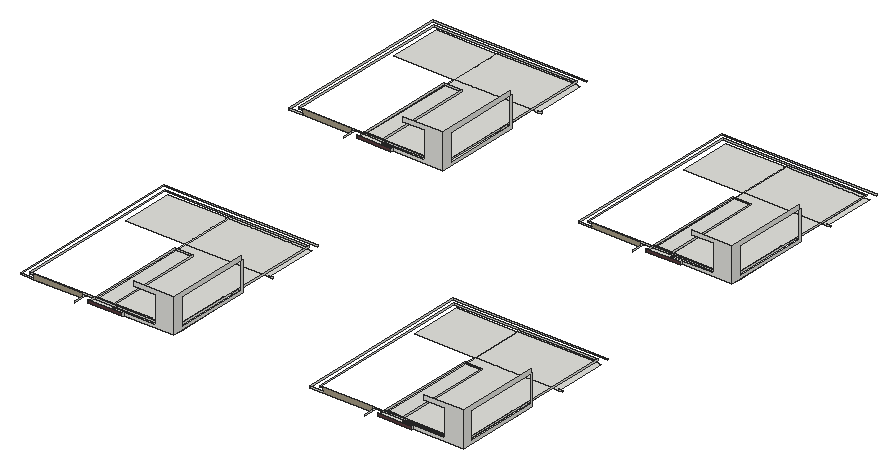
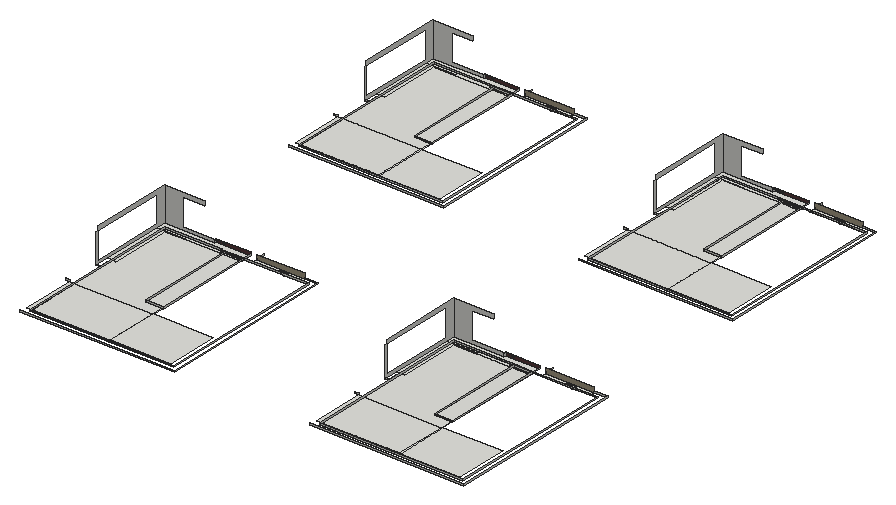
# SketchUp Ruby script. Lengths in inches.
U = 1.inch
M = Sketchup.active_model
def pt(a) = Geom::Point3d.new(a.map { |v| v * U })
def face(e, loops, mat)
  f = e.add_face(loops[0].map { |a| pt(a) })
  loops[1..].each { |l| e.add_face(l.map { |a| pt(a) }).erase! }
  f.material = f.back_material = mat if mat
  f
end
# faces: each face lists its corners as indices into pts; further lists are holes
def faces(e, pts, list, mat = nil) = list.each { |f| face(e, (f[0].is_a?(Array) ? f : [f]).map { |l| l.map { |i| pts[i] } }, mat) }
# xy, xz, yz: faces in a plane at the given z, y or x. An outline is a flat list of corners, or four numbers for a rectangle; further outlines are holes
def ring(l) = l.size == 4 ? [[l[0], l[1]], [l[2], l[1]], [l[2], l[3]], [l[0], l[3]]] : l.each_slice(2).to_a
def flat(e, list, mat, &to3) = list.each { |f| face(e, (f[0].is_a?(Array) ? f : [f]).map { |l| ring(l).map { |u, v| to3.(u, v) } }, mat) }
def xy(e, z, list, mat = nil) = flat(e, list, mat) { |x, y| [x, y, z] }
def xz(e, y, list, mat = nil) = flat(e, list, mat) { |x, z| [x, y, z] }
def yz(e, x, list, mat = nil) = flat(e, list, mat) { |y, z| [x, y, z] }
def lines(e, pts, list) = list.each { |a, b| e.add_line(pt(pts[a]), pt(pts[b])) }
# prism: a flat outline (further loops are holes) pulled along v
def prism(e, loops, v, mat = nil)
  f = face(e, loops, mat); d = Geom::Vector3d.new(v.map { |x| x * U })
  f.pushpull(f.normal.samedirection?(d) ? d.length : -d.length)
end
def box(e, o, s, mat = nil) = prism(e, [[o, [o[0] + s[0], o[1], o[2]], [o[0] + s[0], o[1] + s[1], o[2]], [o[0], o[1] + s[1], o[2]]]], [0, 0, s[2]], mat)
def at(x, y, z, deg = 0) = Geom::Transformation.translation(pt([x, y, z])) * Geom::Transformation.rotation(ORIGIN, Z_AXIS, deg.degrees)
def axes(o, x, y, z) = Geom::Transformation.new([*x, 0, *y, 0, *z, 0, *pt(o).to_a, 1])
def part(name) = M.definitions.add(name)
# library, detail: a bought-in or finely detailed component or shape, given as its bounding box
def library(name, o, s) = part(name).tap { |d| box(d.entities, o, s) }
def detail(e, o, s) = box(e.add_group.entities, o, s)
def put(e, d, t, mat = nil) = e.add_instance(d, t).tap { |i| i.material = mat if mat }
def group(e, t, mat = nil) = e.add_group.tap { |g| g.transformation = t; g.material = mat if mat }.entities
root = M.entities
M.materials.add("[Concrete Tile]").color = [165, 155, 133]
M.materials.add("[Granite Brown]").color = [89, 59, 61]
xy(root,504,[[557.88,1788.5,557.88,1822.9375,890.875,1822.9375,890.875,1835.1875,913.875,1835.1875,913.875,1795.6875,701.53,1795.6875,701.53,1788.5],[1776.07,1788.5,1776.07,1822.9375,2109.0625,1822.9375,2109.0625,1835.1875,2132.0625,1835.1875,2132.0625,1795.6875,1919.71,1795.6875,1919.71,1788.5],[319.53,1799.9375,319.53,1822.9375,401.14,1822.9375,401.14,1806.5625,431.33,1806.5625,431.33,1822.9375,523.04,1822.9375,523.04,1799.9375],[1537.72,1799.9375,1537.72,1822.9375,1619.33,1822.9375,1619.33,1806.5625,1649.52,1806.5625,1649.52,1822.9375,1741.23,1822.9375,1741.23,1799.9375],[557.4,1822.9375,557.4,1827.68,556.44,1827.91,555.39,1823.41],
  [557.4,1822.9375,557.88,1825,557.88,1827.4375,557.4,1827.4375],[650.48,1822.9375,890.875,1822.9375,890.875,1835.1875,784.3125,1835.1875,784.3125,1837.8125,632.49,1837.8125,632.49,1827.4375,650.48,1827.4375],[648.79,1822.9375,650.48,1827.4375],[1775.59,1822.9375,1775.59,1827.68,1774.63,1827.91,1773.58,1823.41],[1775.59,1822.9375,1776.07,1825,1776.07,1827.4375,1775.59,1827.4375],
  [1868.66,1822.9375,2109.0625,1822.9375,2109.0625,1835.1875,2002.5,1835.1875,2002.5,1837.8125,1850.67,1837.8125,1850.67,1827.4375,1868.66,1827.4375],[1866.98,1822.9375,1868.66,1827.4375],[557.88,1825,558.45,1827.4375,557.88,1827.4375],[1776.07,1825,1776.64,1827.4375,1776.07,1827.4375],[557.4,1827.4375,557.88,1827.4375,557.88,1827.57,557.4,1827.68],
  [557.88,1827.4375,558.45,1827.4375,557.88,1827.57],[558.45,1827.4375,558.96,1829.625,557.88,1829.625,557.88,1827.57],[558.45,1827.4375,558.96,1829.625,560,1829.625,560,1827.4375],[560,1827.4375,564.5,1829.625],[564.5,1827.4375,632.49,1829.625],
  [1775.59,1827.4375,1776.07,1827.4375,1776.07,1827.57,1775.59,1827.68],[1776.07,1827.4375,1776.64,1827.4375,1776.07,1827.57],[1776.64,1827.4375,1777.15,1829.625,1776.07,1829.625,1776.07,1827.57],[1776.64,1827.4375,1777.15,1829.625,1778.1875,1829.625,1778.1875,1827.4375],[1778.1875,1827.4375,1782.6875,1829.625],
  [1782.6875,1827.4375,1850.67,1829.625],[557.88,1827.57,557.88,1827.68,557.4,1827.68],[1776.07,1827.57,1776.07,1827.68,1775.59,1827.68],[557.4,1827.68,557.4,1829.99,556.96,1830.09,556.44,1827.91],[1775.59,1827.68,1775.59,1829.99,1775.14,1830.09,1774.63,1827.91],
  [557.4,1829.625,557.88,1829.625,557.88,1829.875,557.4,1829.99],[557.88,1829.625,557.88,1829.875,558.96,1829.625],[558.96,1829.625,557.88,1829.875,557.88,1834.0625,557.99,1834.53,560,1834.0625],[558.96,1829.625,560,1834.0625,560,1829.625],[560,1829.625,564.5,1834.0625],
  [564.5,1829.625,632.49,1837.8125],[1775.59,1829.625,1776.07,1829.625,1776.07,1829.875,1775.59,1829.99],[1776.07,1829.625,1776.07,1829.875,1777.15,1829.625],[1777.15,1829.625,1776.07,1829.875,1776.07,1834.0625,1776.18,1834.53,1778.1875,1834.0625],[1777.15,1829.625,1778.1875,1834.0625,1778.1875,1829.625],
  [1778.1875,1829.625,1782.6875,1834.0625],[1782.6875,1829.625,1850.67,1837.8125],[557.4,1829.99,557.4,1832,556.96,1830.09],[1775.59,1829.99,1775.59,1832,1775.14,1830.09],[557.4,1832,557.88,1834.0625,557.88,1832],
  [557.4,1832,557.88,1834.0625,557.88,1837.8125,557.4,1837.8125],[1775.59,1832,1776.07,1834.0625,1776.07,1832],[1775.59,1832,1776.07,1834.0625,1776.07,1837.8125,1775.59,1837.8125],[557.88,1834.0625,557.88,1837.8125,560,1837.8125,560,1834.0625,557.99,1834.53],[560,1834.0625,564.5,1837.8125],
  [1776.07,1834.0625,1776.07,1837.8125,1778.1875,1837.8125,1778.1875,1834.0625,1776.18,1834.53],[1778.1875,1834.0625,1782.6875,1837.8125],[784.3125,1835.1875,890.875,1835.1875,890.875,2095.79,878.5625,2095.79,878.5625,1837.8125,784.3125,1837.8125],[890.875,1835.1875,913.875,2095.79],[2002.5,1835.1875,2109.0625,1835.1875,2109.0625,2095.79,2096.75,2095.79,2096.75,1837.8125,2002.5,1837.8125],
  [2109.0625,1835.1875,2132.0625,2095.79],[557.4,1837.8125,560,2246.6875],[560,1837.8125,564.5,1838.5625],[564.5,1837.8125,632.49,2246.6875],[632.49,1837.8125,878.5625,1837.8125,878.5625,2095.79,890.875,2095.79,890.875,2295.875,564.5,2295.875,564.5,2246.6875,632.49,2246.6875],
  [1775.59,1837.8125,1778.1875,2246.6875],[1778.1875,1837.8125,1782.6875,1838.5625],[1782.6875,1837.8125,1850.67,2246.6875],[1850.67,1837.8125,2096.75,1837.8125,2096.75,2095.79,2109.0625,2095.79,2109.0625,2295.875,1782.6875,2295.875,1782.6875,2246.6875,1850.67,2246.6875],[560,1838.5625,564.5,2246.6875],
  [1778.1875,1838.5625,1782.6875,2246.6875],[560,2246.6875,564.5,2295.875],[1778.1875,2246.6875,1782.6875,2295.875],[308.87,2295.875,560,2518.89],[560,2295.875,564.5,2518.89],
  [564.5,2295.875,890.875,2518.89],[890.875,2295.875,913.875,2518.89],[1527.06,2295.875,1778.1875,2518.89],[1778.1875,2295.875,1782.6875,2518.89],[1782.6875,2295.875,2109.0625,2518.89],
  [2109.0625,2295.875,2132.0625,2518.89],[560,2518.89,564.5,2531.375],[564.5,2518.89,890.875,2531.375],[1778.1875,2518.89,1782.6875,2531.375],[1782.6875,2518.89,2109.0625,2531.375],
  [557.88,3203.1875,557.88,3237.625,890.875,3237.625,890.875,3249.875,913.875,3249.875,913.875,3210.375,701.53,3210.375,701.53,3203.1875],[1776.07,3203.1875,1776.07,3237.625,2109.0625,3237.625,2109.0625,3249.875,2132.0625,3249.875,2132.0625,3210.375,1919.71,3210.375,1919.71,3203.1875],[319.53,3214.625,319.53,3237.625,401.14,3237.625,401.14,3221.25,431.33,3221.25,431.33,3237.625,523.04,3237.625,523.04,3214.625],[1537.72,3214.625,1537.72,3237.625,1619.33,3237.625,1619.33,3221.25,1649.52,3221.25,1649.52,3237.625,1741.23,3237.625,1741.23,3214.625],[557.4,3237.625,557.4,3242.37,556.44,3242.59,555.39,3238.09],
  [557.4,3237.625,557.88,3239.6875,557.88,3242.125,557.4,3242.125],[650.48,3237.625,890.875,3237.625,890.875,3249.875,784.3125,3249.875,784.3125,3252.5,632.49,3252.5,632.49,3242.125,650.48,3242.125],[648.79,3237.625,650.48,3242.125],[1775.59,3237.625,1775.59,3242.37,1774.63,3242.59,1773.58,3238.09],[1775.59,3237.625,1776.07,3239.6875,1776.07,3242.125,1775.59,3242.125],
  [1868.66,3237.625,2109.0625,3237.625,2109.0625,3249.875,2002.5,3249.875,2002.5,3252.5,1850.67,3252.5,1850.67,3242.125,1868.66,3242.125],[1866.98,3237.625,1868.66,3242.125],[557.88,3239.6875,558.45,3242.125,557.88,3242.125],[1776.07,3239.6875,1776.64,3242.125,1776.07,3242.125],[557.4,3242.125,557.88,3242.125,557.88,3242.26,557.4,3242.37],
  [557.88,3242.125,558.45,3242.125,557.88,3242.26],[558.45,3242.125,558.96,3244.3125,557.88,3244.3125,557.88,3242.26],[558.45,3242.125,558.96,3244.3125,560,3244.3125,560,3242.125],[560,3242.125,564.5,3244.3125],[564.5,3242.125,632.49,3244.3125],
  [1775.59,3242.125,1776.07,3242.125,1776.07,3242.26,1775.59,3242.37],[1776.07,3242.125,1776.64,3242.125,1776.07,3242.26],[1776.64,3242.125,1777.15,3244.3125,1776.07,3244.3125,1776.07,3242.26],[1776.64,3242.125,1777.15,3244.3125,1778.1875,3244.3125,1778.1875,3242.125],[1778.1875,3242.125,1782.6875,3244.3125],
  [1782.6875,3242.125,1850.67,3244.3125],[557.88,3242.26,557.88,3242.37,557.4,3242.37],[1776.07,3242.26,1776.07,3242.37,1775.59,3242.37],[557.4,3242.37,557.4,3244.68,556.96,3244.78,556.44,3242.59],[1775.59,3242.37,1775.59,3244.68,1775.14,3244.78,1774.63,3242.59],
  [557.4,3244.3125,557.88,3244.3125,557.88,3244.5625,557.4,3244.68],[557.88,3244.3125,557.88,3244.5625,558.96,3244.3125],[558.96,3244.3125,557.88,3244.5625,557.88,3248.75,557.99,3249.22,560,3248.75],[558.96,3244.3125,560,3248.75,560,3244.3125],[560,3244.3125,564.5,3248.75],
  [564.5,3244.3125,632.49,3252.5],[1775.59,3244.3125,1776.07,3244.3125,1776.07,3244.5625,1775.59,3244.68],[1776.07,3244.3125,1776.07,3244.5625,1777.15,3244.3125],[1777.15,3244.3125,1776.07,3244.5625,1776.07,3248.75,1776.18,3249.22,1778.1875,3248.75],[1777.15,3244.3125,1778.1875,3248.75,1778.1875,3244.3125],
  [1778.1875,3244.3125,1782.6875,3248.75],[1782.6875,3244.3125,1850.67,3252.5],[557.4,3244.68,557.4,3246.6875,556.96,3244.78],[1775.59,3244.68,1775.59,3246.6875,1775.14,3244.78],[557.4,3246.6875,557.88,3248.75,557.88,3246.6875],
  [557.4,3246.6875,557.88,3248.75,557.88,3252.5,557.4,3252.5],[1775.59,3246.6875,1776.07,3248.75,1776.07,3246.6875],[1775.59,3246.6875,1776.07,3248.75,1776.07,3252.5,1775.59,3252.5],[557.88,3248.75,557.88,3252.5,560,3252.5,560,3248.75,557.99,3249.22],[560,3248.75,564.5,3252.5],
  [1776.07,3248.75,1776.07,3252.5,1778.1875,3252.5,1778.1875,3248.75,1776.18,3249.22],[1778.1875,3248.75,1782.6875,3252.5],[784.3125,3249.875,890.875,3249.875,890.875,3510.48,878.5625,3510.48,878.5625,3252.5,784.3125,3252.5],[890.875,3249.875,913.875,3510.48],[2002.5,3249.875,2109.0625,3249.875,2109.0625,3510.48,2096.75,3510.48,2096.75,3252.5,2002.5,3252.5],
  [2109.0625,3249.875,2132.0625,3510.48],[557.4,3252.5,560,3661.375],[560,3252.5,564.5,3253.25],[564.5,3252.5,632.49,3661.375],[632.49,3252.5,878.5625,3252.5,878.5625,3510.48,890.875,3510.48,890.875,3710.5625,564.5,3710.5625,564.5,3661.375,632.49,3661.375],
  [1775.59,3252.5,1778.1875,3661.375],[1778.1875,3252.5,1782.6875,3253.25],[1782.6875,3252.5,1850.67,3661.375],[1850.67,3252.5,2096.75,3252.5,2096.75,3510.48,2109.0625,3510.48,2109.0625,3710.5625,1782.6875,3710.5625,1782.6875,3661.375,1850.67,3661.375],[560,3253.25,564.5,3661.375],
  [1778.1875,3253.25,1782.6875,3661.375],[560,3661.375,564.5,3710.5625],[1778.1875,3661.375,1782.6875,3710.5625],[308.87,3710.5625,560,3933.57],[560,3710.5625,564.5,3933.57],
  [564.5,3710.5625,890.875,3933.57],[890.875,3710.5625,913.875,3933.57],[1527.06,3710.5625,1778.1875,3933.57],[1778.1875,3710.5625,1782.6875,3933.57],[1782.6875,3710.5625,2109.0625,3933.57],
  [2109.0625,3710.5625,2132.0625,3933.57],[560,3933.57,564.5,3946.0625],[564.5,3933.57,890.875,3946.0625],[1778.1875,3933.57,1782.6875,3946.0625],[1782.6875,3933.57,2109.0625,3946.0625]])
xy(root,504,[[557.4,1788.5,557.88,1822.9375],[1775.59,1788.5,1776.07,1822.9375],[557.4,1822.9375,557.88,1822.9375,557.88,1825],[1775.59,1822.9375,1776.07,1822.9375,1776.07,1825],[557.4,1827.68,557.88,1829.625],
  [1775.59,1827.68,1776.07,1829.625],[557.88,1829.875,557.4,1829.99,557.88,1829.99],[1776.07,1829.875,1775.59,1829.99,1776.07,1829.99],[557.4,1829.99,557.88,1832],[1775.59,1829.99,1776.07,1832],
  [1775.59,1832,1776.07,1832,1776.07,1834.0625],[557.4,3203.1875,557.88,3237.625],[1775.59,3203.1875,1776.07,3237.625],[557.4,3237.625,557.88,3237.625,557.88,3239.6875],[1775.59,3237.625,1776.07,3237.625,1776.07,3239.6875],
  [557.4,3242.37,557.88,3244.3125],[1775.59,3242.37,1776.07,3244.3125],[557.88,3244.5625,557.4,3244.68,557.88,3244.68],[1776.07,3244.5625,1775.59,3244.68,1776.07,3244.68],[557.4,3244.68,557.88,3246.6875],
  [1775.59,3244.68,1776.07,3246.6875]],"[Granite Brown]")
xz(root,1788.5,[[557.4,504,557.88,510],[557.88,504,701.53,516.375],[1775.59,504,1776.07,510],[1776.07,504,1919.71,516.375]],"[Granite Brown]")
xz(root,1795.6875,[[701.53,504,913.875,504,913.875,648.6875,745.8,648.6875,745.8,630,835.99,630,835.99,517.25,657.21,517.25,657.21,516.375,701.53,516.375],[1919.71,504,2132.0625,504,2132.0625,648.6875,1963.98,648.6875,1963.98,630,2054.17,630,2054.17,517.25,1875.4,517.25,1875.4,516.375,1919.71,516.375]])
xz(root,1799.9375,[[262.875,504,319.53,510],[1481.0625,504,1537.72,510]])
xz(root,1799.9375,[[319.53,504,523.04,525.4375],[1537.72,504,1741.23,525.4375]],"[Concrete Tile]")
xz(root,1822.9375,[[285.875,504,285.875,510,557.4,510,557.4,504,401.14,504,386.33,504.07,386.33,504],[386.33,504,386.33,504.07,401.14,504],[557.4,504,648.79,510],[648.79,504,650.48,510],[650.48,504,890.875,510],
  [1504.0625,504,1504.0625,510,1775.59,510,1775.59,504,1619.33,504,1604.52,504.07,1604.52,504],[1604.52,504,1604.52,504.07,1619.33,504],[1775.59,504,1866.98,510],[1866.98,504,1868.66,510],[1868.66,504,2109.0625,510]])
xz(root,1827.4375,[[557.4,504,632.49,510],[632.49,504,648.79,510],[648.79,504,650.48,510],[1775.59,504,1850.67,510],[1850.67,504,1866.98,510],
  [1866.98,504,1868.66,510]])
xz(root,1829.625,[[557.4,504,632.49,510],[1775.59,504,1850.67,510]])
xz(root,2156.01,[[894.3125,504,913.875,510],[2112.5,504,2132.0625,510]])
xz(root,2246.6875,[[557.4,504,632.49,510],[1775.59,504,1850.67,510]])
xz(root,2295.875,[[913.875,504,930.75,510],[2132.0625,504,2148.9375,510]])
xz(root,2531.375,[[285.875,504,890.875,510],[1504.0625,504,2109.0625,510]])
xz(root,2554.375,[[262.875,504,913.875,510],[1481.0625,504,2132.0625,510]])
xz(root,3203.1875,[[557.4,504,557.88,510],[557.88,504,701.53,516.375],[1775.59,504,1776.07,510],[1776.07,504,1919.71,516.375]],"[Granite Brown]")
xz(root,3210.375,[[701.53,504,913.875,504,913.875,648.6875,745.8,648.6875,745.8,630,835.99,630,835.99,517.25,657.21,517.25,657.21,516.375,701.53,516.375],[1919.71,504,2132.0625,504,2132.0625,648.6875,1963.98,648.6875,1963.98,630,2054.17,630,2054.17,517.25,1875.4,517.25,1875.4,516.375,1919.71,516.375]])
xz(root,3214.625,[[262.875,504,319.53,510],[1481.0625,504,1537.72,510]])
xz(root,3214.625,[[319.53,504,523.04,525.4375],[1537.72,504,1741.23,525.4375]],"[Concrete Tile]")
xz(root,3237.625,[[285.875,504,285.875,510,557.4,510,557.4,504,401.14,504,386.33,504.07,386.33,504],[386.33,504,386.33,504.07,401.14,504],[557.4,504,648.79,510],[648.79,504,650.48,510],[650.48,504,890.875,510],
  [1504.0625,504,1504.0625,510,1775.59,510,1775.59,504,1619.33,504,1604.52,504.07,1604.52,504],[1604.52,504,1604.52,504.07,1619.33,504],[1775.59,504,1866.98,510],[1866.98,504,1868.66,510],[1868.66,504,2109.0625,510]])
xz(root,3242.125,[[557.4,504,632.49,510],[632.49,504,648.79,510],[648.79,504,650.48,510],[1775.59,504,1850.67,510],[1850.67,504,1866.98,510],
  [1866.98,504,1868.66,510]])
xz(root,3244.3125,[[557.4,504,632.49,510],[1775.59,504,1850.67,510]])
xz(root,3570.7,[[894.3125,504,913.875,510],[2112.5,504,2132.0625,510]])
xz(root,3661.375,[[557.4,504,632.49,510],[1775.59,504,1850.67,510]])
xz(root,3710.5625,[[913.875,504,930.75,510],[2132.0625,504,2148.9375,510]])
xz(root,3946.0625,[[285.875,504,890.875,510],[1504.0625,504,2109.0625,510]])
xz(root,3969.0625,[[262.875,504,913.875,510],[1481.0625,504,2132.0625,510]])
yz(root,262.875,[[1799.9375,504,2554.375,510],[3214.625,504,3969.0625,510]])
yz(root,285.875,[[1822.9375,504,2531.375,510],[3237.625,504,3946.0625,510]])
yz(root,523.04,[[1763.25,504,1799.9375,510],[3177.9375,504,3214.625,510]])
yz(root,557.4,[[1788.5,504,1822.9375,510],[1822.9375,504,1827.4375,510],[1827.4375,504,1829.625,510],[1829.625,504,2246.6875,510],[3203.1875,504,3237.625,510],
  [3237.625,504,3242.125,510],[3242.125,504,3244.3125,510],[3244.3125,504,3661.375,510]])
yz(root,632.49,[[1827.4375,504,1829.625,510],[1829.625,504,2246.6875,510],[3242.125,504,3244.3125,510],[3244.3125,504,3661.375,510]])
yz(root,648.79,[[1822.9375,504,1827.4375,510],[3237.625,504,3242.125,510]])
yz(root,650.48,[[1822.9375,504,1827.4375,510],[3237.625,504,3242.125,510]])
yz(root,701.53,[[1788.5,504,1795.6875,516.375],[3203.1875,504,3210.375,516.375]])
yz(root,890.875,[[1822.9375,504,2531.375,510],[3237.625,504,3946.0625,510]])
yz(root,894.3125,[[2124.51,504,2156.01,510],[3539.2,504,3570.7,510]])
yz(root,913.875,[[1795.6875,504,2156.01,504,2156.01,630,2148.83,630,2148.83,517.25,1835.1875,517.25,1835.1875,630,2148.83,630,2148.83,648.6875,1795.6875,648.6875],[3210.375,504,3570.7,504,3570.7,630,3563.51,630,3563.51,517.25,3249.875,517.25,3249.875,630,3563.51,630,3563.51,648.6875,3210.375,648.6875]])
yz(root,1481.0625,[[1799.9375,504,2554.375,510],[3214.625,504,3969.0625,510]])
yz(root,1504.0625,[[1822.9375,504,2531.375,510],[3237.625,504,3946.0625,510]])
yz(root,1741.23,[[1763.25,504,1799.9375,510],[3177.9375,504,3214.625,510]])
yz(root,1775.59,[[1788.5,504,1822.9375,510],[1822.9375,504,1827.4375,510],[1827.4375,504,1829.625,510],[1829.625,504,2246.6875,510],[3203.1875,504,3237.625,510],
  [3237.625,504,3242.125,510],[3242.125,504,3244.3125,510],[3244.3125,504,3661.375,510]])
yz(root,1850.67,[[1827.4375,504,1829.625,510],[1829.625,504,2246.6875,510],[3242.125,504,3244.3125,510],[3244.3125,504,3661.375,510]])
yz(root,1866.98,[[1822.9375,504,1827.4375,510],[3237.625,504,3242.125,510]])
yz(root,1868.66,[[1822.9375,504,1827.4375,510],[3237.625,504,3242.125,510]])
yz(root,1919.71,[[1788.5,504,1795.6875,516.375],[3203.1875,504,3210.375,516.375]])
yz(root,2109.0625,[[1822.9375,504,2531.375,510],[3237.625,504,3946.0625,510]])
yz(root,2112.5,[[2124.51,504,2156.01,510],[3539.2,504,3570.7,510]])
yz(root,2132.0625,[[1795.6875,504,2156.01,504,2156.01,630,2148.83,630,2148.83,517.25,1835.1875,517.25,1835.1875,630,2148.83,630,2148.83,648.6875,1795.6875,648.6875],[3210.375,504,3570.7,504,3570.7,630,3563.51,630,3563.51,517.25,3249.875,517.25,3249.875,630,3563.51,630,3563.51,648.6875,3210.375,648.6875]])
p = [[401.14,1806.5625,504],[401.14,1822.9375,504],[386.33,1822.9375,504.07],[386.33,1806.5625,504.07],[1619.33,1806.5625,504],[1619.33,1822.9375,504],
  [1604.52,1822.9375,504.07],[1604.52,1806.5625,504.07],[401.14,3221.25,504],[401.14,3237.625,504],[386.33,3237.625,504.07],[386.33,3221.25,504.07],
  [1619.33,3221.25,504],[1619.33,3237.625,504],[1604.52,3237.625,504.07],[1604.52,3221.25,504.07],[1741.23,1778.3125,504],[1741.23,1778.3125,510],
  [523.04,1778.3125,504],[523.04,1778.3125,510],[1741.23,3193,504],[1741.23,3193,510],[523.04,3193,504],[523.04,3193,510]]
faces(root,p,[[0,1,2,3],[4,5,6,7],[8,9,10,11],[12,13,14,15]])
lines(root,p,[[16,17],[18,19],[20,21],[22,23]])
